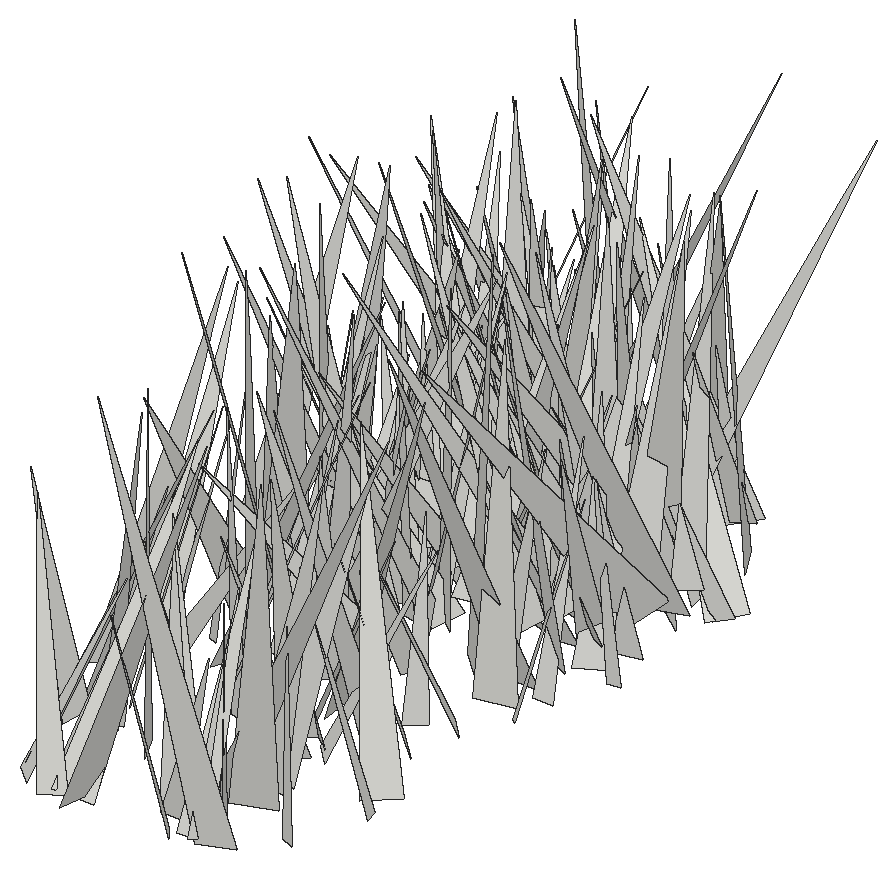
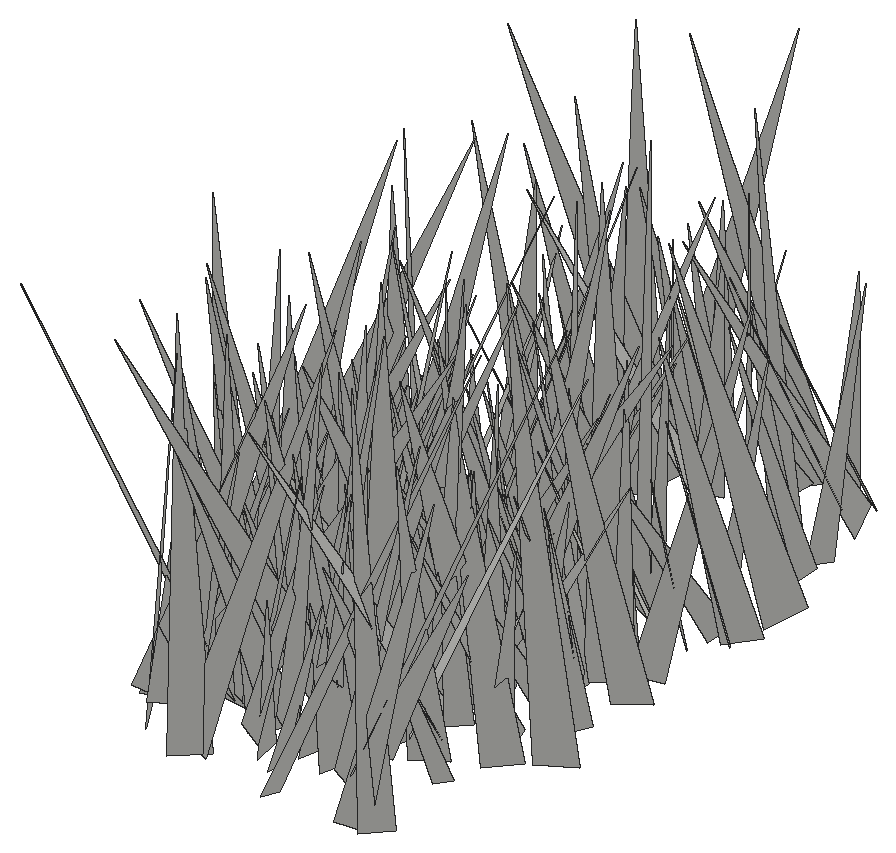
# SketchUp Ruby script. Lengths in inches.
U = 1.inch
M = Sketchup.active_model
def pt(a) = Geom::Point3d.new(a.map { |v| v * U })
def face(e, loops, mat)
  f = e.add_face(loops[0].map { |a| pt(a) })
  loops[1..].each { |l| e.add_face(l.map { |a| pt(a) }).erase! }
  f.material = f.back_material = mat if mat
  f
end
# faces: each face lists its corners as indices into pts; further lists are holes
def faces(e, pts, list, mat = nil) = list.each { |f| face(e, (f[0].is_a?(Array) ? f : [f]).map { |l| l.map { |i| pts[i] } }, mat) }
# xy, xz, yz: faces in a plane at the given z, y or x. An outline is a flat list of corners, or four numbers for a rectangle; further outlines are holes
def ring(l) = l.size == 4 ? [[l[0], l[1]], [l[2], l[1]], [l[2], l[3]], [l[0], l[3]]] : l.each_slice(2).to_a
def flat(e, list, mat, &to3) = list.each { |f| face(e, (f[0].is_a?(Array) ? f : [f]).map { |l| ring(l).map { |u, v| to3.(u, v) } }, mat) }
def xy(e, z, list, mat = nil) = flat(e, list, mat) { |x, y| [x, y, z] }
def xz(e, y, list, mat = nil) = flat(e, list, mat) { |x, z| [x, y, z] }
def yz(e, x, list, mat = nil) = flat(e, list, mat) { |y, z| [x, y, z] }
def lines(e, pts, list) = list.each { |a, b| e.add_line(pt(pts[a]), pt(pts[b])) }
# prism: a flat outline (further loops are holes) pulled along v
def prism(e, loops, v, mat = nil)
  f = face(e, loops, mat); d = Geom::Vector3d.new(v.map { |x| x * U })
  f.pushpull(f.normal.samedirection?(d) ? d.length : -d.length)
end
def box(e, o, s, mat = nil) = prism(e, [[o, [o[0] + s[0], o[1], o[2]], [o[0] + s[0], o[1] + s[1], o[2]], [o[0], o[1] + s[1], o[2]]]], [0, 0, s[2]], mat)
def at(x, y, z, deg = 0) = Geom::Transformation.translation(pt([x, y, z])) * Geom::Transformation.rotation(ORIGIN, Z_AXIS, deg.degrees)
def axes(o, x, y, z) = Geom::Transformation.new([*x, 0, *y, 0, *z, 0, *pt(o).to_a, 1])
def part(name) = M.definitions.add(name)
# library, detail: a bought-in or finely detailed component or shape, given as its bounding box
def library(name, o, s) = part(name).tap { |d| box(d.entities, o, s) }
def detail(e, o, s) = box(e.add_group.entities, o, s)
def put(e, d, t, mat = nil) = e.add_instance(d, t).tap { |i| i.material = mat if mat }
def group(e, t, mat = nil) = e.add_group.tap { |g| g.transformation = t; g.material = mat if mat }.entities
root = M.entities
c1 = part("fur_instance\#9")
p = [[0.8125,0,1.79],[0.67,-0.02,1.48],[0,-0.11,0],[0,0.11,0]]
faces(c1.entities,p,[[0,1,2,3]])
put(root,c1,axes([145.41,167.63,-28.22],[-0.98581,-7.65367,2.64082],[-7.9173,0.35473,-1.92744],[-1.69382,2.79641,7.47232]))
put(root,c1,axes([143.71,167.37,-28.22],[-3.00946,-2.45302,0.73779],[-2.54129,3.00205,-0.38468],[0.32167,0.76736,3.86344]))
put(root,c1,axes([140.13,167.29,-28.22],[7.76844,-0.71206,0.72464],[-0.74639,-7.79129,0.34557],[-0.68922,0.41169,7.79335]))
put(root,c1,axes([143.16,168.27,-28.22],[1.4619,-3.63585,0.57448],[-3.60479,-1.28901,1.01518],[0.74496,0.89757,3.78497]))
put(root,c1,axes([139.28,167.01,-28.22],[-1.32199,4.73147,0.88748],[4.77716,1.17578,0.84759],[-0.59431,-1.0737,4.83901]))
put(root,c1,axes([137.77,167.43,-28.22],[2.47782,3.1575,0.0552],[3.13992,-2.45577,-0.47176],[0.33732,-0.3344,3.98583]))
put(root,c1,axes([142.86,168.82,-28.22],[1.68942,-4.24341,1.91691],[-4.60334,-1.82876,0.00876],[-0.70022,1.78447,4.56734]))
put(root,c1,axes([144.73,167.74,-28.22],[3.50267,-1.34823,2.1537],[-1.97697,-3.75014,0.86764],[-1.59615,1.68627,3.65152]))
put(root,c1,axes([144.74,170.4,-28.22],[3.4393,-6.56896,1.063],[-6.65437,-3.3911,0.57422],[0.02233,1.20797,7.39258]))
put(root,c1,axes([144.92,168.69,-28.22],[3.08289,1.97486,1.70839],[2.08981,-3.45082,0.21788],[-1.56569,-0.71742,3.6547]))
put(root,c1,axes([144.52,167.62,-28.22],[-1.16488,5.07104,1.08343],[5.11451,1.30667,-0.61696],[0.85504,-0.90739,5.16641]))
put(root,c1,axes([138.8,167.92,-28.22],[2.95968,3.81178,0.17357],[3.80838,-2.96454,0.16477],[-0.23661,-0.0359,4.82309]))
put(root,c1,axes([139.86,167.31,-28.22],[-2.51338,5.74575,1.01303],[5.46798,2.70448,-1.77311],[2.03497,-0.17044,6.01555]))
put(root,c1,axes([138.6,170.6,-28.22],[6.91292,1.02767,1.79019],[1.3308,-7.00178,-1.11957],[-1.57792,-1.40299,6.89863]))
put(root,c1,axes([147.02,169.24,-28.22],[1.49909,3.09185,1.25062],[3.12666,-1.78006,0.6529],[-1.16087,-0.8017,3.3735]))
put(root,c1,axes([142.28,170.18,-28.22],[1.59272,-3.9303,2.28796],[-4.37909,-1.9795,-0.352],[-1.22702,1.96293,4.22612]))
put(root,c1,axes([143.78,169.98,-28.22],[7.97011,-1.5942,0.50435],[-1.65185,-7.88792,1.1707],[-0.25934,1.24806,8.04323]))
put(root,c1,axes([136.72,171.46,-28.22],[4.20178,-1.75309,2.00996],[-1.5081,-4.65512,-0.90755],[-2.19975,-0.15714,4.46146]))
put(root,c1,axes([144.19,171.61,-28.22],[1.87666,-6.19619,1.68038],[-6.32701,-1.4881,1.57887],[1.08876,2.03251,6.27868]))
put(root,c1,axes([137.36,168.47,-28.22],[6.20269,2.14266,0.41588],[1.88774,-5.89525,2.21806],[-1.09562,1.97291,6.17613]))
put(root,c1,axes([137.88,171.68,-28.22],[2.52401,-3.24586,0.70539],[-3.32076,-2.44552,0.62916],[0.07602,0.94215,4.0633]))
put(root,c1,axes([139.83,171.2,-28.22],[5.01686,3.02729,2.73746],[3.17963,-5.61852,0.38618],[-2.55892,-1.04628,5.84673]))
put(root,c1,axes([148.0625,172.21,-28.22],[-3.92472,-1.58946,0.29836],[-1.61245,3.78584,-1.04222],[-0.12416,1.07696,4.10409]))
put(root,c1,axes([144.14,172.34,-28.22],[0.67083,5.9533,2.27987],[6.17356,-0.03505,-1.72498],[1.58958,-2.37626,5.73727]))
put(root,c1,axes([136.5625,172.31,-28.22],[4.46137,-0.22154,0.62784],[-0.29219,-4.4737,0.49769],[-0.59824,0.53291,4.43905]))
put(root,c1,axes([143.04,174.73,-28.22],[3.50702,-4.68842,0.88051],[-4.69288,-3.58696,-0.4079],[-0.85643,0.45629,5.84073]))
put(root,c1,axes([141.98,170.6,-28.22],[5.9455,4.2001,0.21568],[4.05072,-5.81939,1.66213],[-1.13095,1.23699,7.08711]))
put(root,c1,axes([144.01,173.83,-28.22],[-1.49858,-3.44059,1.04989],[-3.40031,0.98374,-1.62968],[-1.17382,1.54281,3.38047]))
put(root,c1,axes([137.58,175.24,-28.22],[-3.46561,0.71078,2.1355],[1.4755,3.67824,1.17025],[1.69955,-1.74395,3.33859]))
put(root,c1,axes([147.625,173.29,-28.22],[2.97491,-4.25566,3.74848],[-5.0806,-3.88069,-0.37363],[-2.51977,2.80026,5.17891]))
put(root,c1,axes([145.67,175.61,-28.22],[-0.89834,-6.55906,1.37521],[-6.65422,0.70817,-0.96916],[-0.7961,1.48213,6.54897]))
put(root,c1,axes([137.35,173.47,-28.22],[4.69542,3.0157,0.91715],[3.05189,-4.76105,0.03053],[-0.78841,-0.46959,5.58037]))
put(root,c1,axes([146.1,176.49,-28.22],[-3.15103,-4.03715,0.66571],[-3.75697,3.18756,1.54769],[1.62077,-0.46003,4.88182]))
put(root,c1,axes([140.88,174.49,-28.22],[1.89742,4.59885,2.05217],[4.78177,-2.33318,0.8074],[-1.57969,-1.53878,4.90894]))
put(root,c1,axes([144.35,174.39,-28.22],[3.00056,3.161,0.00616],[3.13284,-2.97269,-0.58633],[0.42105,-0.40809,4.31874]))
put(root,c1,axes([143.93,174.89,-28.22],[-6.33694,-5.31771,1.42218],[-5.44687,5.74429,-2.79146],[-0.79519,3.03026,7.78734]))
put(root,c1,axes([142.93,175.65,-28.22],[3.86213,1.08614,0.2172],[1.09096,-3.86634,-0.0646],[-0.19154,-0.12107,4.01143]))
put(root,c1,axes([142.83,177.24,-28.22],[7.51831,-0.309,0.51299],[-0.23256,-7.46002,-1.08516],[-0.55186,-1.06592,7.446]))
put(root,c1,axes([135.35,174.89,-28.22],[6.60662,-2.19065,2.41659],[-2.83754,-6.55209,1.81792],[-1.6085,2.56075,6.71874]))
put(root,c1,axes([139.13,177.43,-28.22],[-3.84702,-6.56229,2.86732],[-6.71624,4.43571,1.14075],[2.48541,1.82909,7.52076]))
put(root,c1,axes([141.31,176.01,-28.22],[2.64561,4.33348,1.24236],[4.47199,-2.70465,-0.08904],[-0.56902,-1.10798,5.07645]))
put(root,c1,axes([146.58,178.38,-28.22],[-3.28468,-3.33783,0.1825],[-3.30088,3.27904,0.56182],[0.52783,-0.26523,4.64915]))
put(root,c1,axes([141.5,178.35,-28.22],[3.06125,-3.87557,0.82155],[-3.90702,-3.12527,-0.1848],[-0.65588,0.52812,4.93529]))
put(root,c1,axes([142.17,180.51,-28.22],[-5.57045,-1.42182,0.3414],[-1.0257,4.7578,3.07884],[1.04215,-2.91715,4.85512]))
put(root,c1,axes([136.34,180.7,-28.22],[5.34512,-3.23236,0.64666],[-2.65449,-4.95104,-2.80671],[-1.95449,-2.11559,5.5804]))
put(root,c1,axes([135.875,177.12,-28.22],[2.95956,2.83712,0.75066],[2.89518,-2.997,-0.08741],[-0.48027,-0.58351,4.09885]))
put(root,c1,axes([145.45,177.71,-28.22],[-2.47,2.58512,1.49197],[2.74392,2.72878,-0.18549],[1.17462,-0.93843,3.57063]))
put(root,c1,axes([136.35,176.99,-28.22],[3.53802,-1.77872,0.68161],[-1.86523,-2.94336,2.00089],[0.38644,2.07817,3.41729]))
put(root,c1,axes([135.49,176.93,-28.22],[-3.09006,5.24053,1.65653],[5.13422,3.43055,-1.27548],[1.9614,-0.72379,5.94851]))
put(root,c1,axes([146.27,181.89,-28.22],[-0.28609,-7.90952,0.17476],[-7.91116,0.28452,-0.07401],[-0.06767,0.17732,7.91434]))
put(root,c1,axes([138.21,177.04,-28.22],[6.82155,0.82248,0.97272],[0.53436,-6.65794,1.88216],[-1.15634,1.77527,6.60814]))
put(root,c1,axes([142.74,181.92,-27.1],[-6.5639,-4.29471,0.69968],[-4.06333,6.50273,1.7952],[1.55674,-1.13527,7.63588]))
put(root,c1,axes([140.64,179.44,-28.22],[6.1687,-0.67373,2.21616],[-0.70194,-6.55164,-0.0379],[-2.20738,0.2006,6.20527]))
put(root,c1,axes([137.01,177.98,-28.22],[2.28996,3.33239,0.84649],[3.03653,-2.43723,1.38011],[-1.61271,0.14282,3.80053]))
put(root,c1,axes([137.1,181.5,-28.22],[5.72891,-5.77899,0.7373],[-5.79412,-5.75966,-0.12335],[-0.60698,0.43635,8.13646]))
put(root,c1,axes([138.19,177.99,-28.22],[3.1839,3.43631,0.24845],[3.39454,-3.18669,0.57383],[-0.5891,0.20968,4.64932]))
put(root,c1,axes([139.12,181.21,-28.22],[2.70621,-3.86796,1.26709],[-3.69816,-2.97221,-1.17466],[-1.70008,0.30833,4.57219]))
put(root,c1,axes([146.53,180.4,-28.22],[-1.49682,6.02983,3.22428],[6.74332,1.8484,-0.32627],[1.1325,-3.03643,6.20426]))
put(root,c1,axes([139.68,180.76,-28.22],[3.87779,-2.1954,0.31482],[-2.2129,-3.78759,0.8446],[0.14815,0.88911,4.37535]))
put(root,c1,axes([143.24,180.38,-28.22],[-3.36679,-6.63148,1.92496],[-6.20382,1.96447,-4.08298],[-3.03226,3.34389,6.21619]))
put(root,c1,axes([138.88,181.55,-27.1],[6.72646,1.81373,2.96578],[2.30607,-7.16166,-0.85049],[-2.60144,-1.65881,6.91459]))
put(root,c1,axes([144.71,181.58,-28.22],[-4.52397,-6.09316,3.51067],[-6.34353,5.33763,1.08955],[3.03497,2.07386,7.51038]))
put(root,c1,axes([140.73,181.74,-28.22],[-7.80525,1.8691,2.4402],[2.24771,8.01322,1.05174],[2.09664,-1.63243,7.95672]))
put(root,c1,axes([139.53,178.46,-28.22],[1.84381,6.83005,0.32521],[6.75707,-1.87158,0.99709],[-1.04756,-0.05069,7.00393]))
put(root,c1,axes([148.02,186.2,-27.1],[5.96387,-5.74764,0.45925],[-4.68382,-5.21453,-4.43673],[-3.36276,-2.93042,6.99418]))
put(root,c1,axes([137.58,182.1875,-28.22],[5.69454,1.71793,1.14191],[1.95584,-5.5622,-1.38552],[-0.6557,-1.67144,5.78441]))
put(root,c1,axes([147.72,179.86,-28.22],[2.63979,2.66437,0.28601],[2.37928,-2.51517,1.47039],[-1.23275,0.85099,3.4504]))
put(root,c1,axes([135.31,183.23,-27.1],[5.21183,-0.69159,1.00189],[-0.40075,-5.13378,-1.45906],[-1.14955,-1.3458,5.051]))
put(root,c1,axes([136.49,181.375,-27.1],[3.11612,2.14822,0.04863],[2.13222,-3.08072,-0.53874],[0.26618,-0.47091,3.74631]))
put(root,c1,axes([145.86,181.5,-28.22],[3.92282,-1.4058,1.44453],[-1.66907,-4.03753,0.60333],[-1.1301,1.0833,4.1232]))
put(root,c1,axes([147.85,181.91,-27.1],[-3.61019,-4.99925,2.09321],[-5.40705,3.49453,-0.97958],[0.37125,2.28107,6.08822]))
put(root,c1,axes([144.81,185.4,-27.1],[-6.99156,-3.62516,0.34789],[-3.32905,6.6672,2.57109],[1.47657,-2.13338,7.444]))
put(root,c1,axes([141.02,186.1,-28.22],[-5.60645,-3.595,0.79099],[-2.74257,5.04084,3.47133],[2.4552,-2.57833,5.68385]))
put(root,c1,axes([139.18,183.02,-28.22],[3.73633,3.15118,1.53756],[3.50493,-3.41917,-1.50964],[-0.09758,-2.15258,4.64878]))
put(root,c1,axes([142.04,183.64,-28.22],[-4.08347,2.98679,1.40676],[3.27171,3.36098,2.36101],[-0.44252,-2.71247,4.47451]))
put(root,c1,axes([142.17,181.43,-27.1],[2.11114,4.26728,1.69749],[4.08085,-2.60007,1.46097],[-2.10662,-0.76029,4.53125]))
put(root,c1,axes([147.66,181.41,-28.22],[0.78964,4.34465,0.57519],[4.335,-0.86018,0.54605],[-0.64386,-0.46311,4.38193]))
put(root,c1,axes([147,184.85,-28.22],[4.67947,-2.49587,0.44393],[-2.29207,-4.56374,-1.49753],[-1.08298,-1.12554,5.08765]))
put(root,c1,axes([138.2,182.58,-28.22],[1.93796,6.92662,2.2466],[6.80944,-0.90011,-3.09877],[2.58009,-2.82714,6.49087]))
put(root,c1,axes([141.64,183.25,-27.1],[5.91305,2.63208,1.30513],[2.84881,-5.85376,-1.10147],[-0.71801,-1.54954,6.37799]))
put(root,c1,axes([141.88,183.62,-28.22],[-3.26006,-5.04679,2.60885],[-5.29814,3.78652,0.70434],[2.05082,1.75965,5.96674]))
put(root,c1,axes([147.875,183.93,-27.1],[-2.11494,-3.26023,0.3236],[-3.25153,2.04149,-0.68318],[-0.40176,0.64034,3.82562]))
put(root,c1,axes([138.71,183.23,-27.1],[4.6292,0.17151,0.50537],[0.17521,-4.6565,-0.02456],[-0.5041,-0.0434,4.63231]))
put(root,c1,axes([140.17,183.61,-28.22],[-0.67807,6.71445,3.30984],[6.96597,-0.65101,2.74773],[-2.74118,-3.31527,6.16389]))
put(root,c1,axes([139.07,182.91,-27.1],[-0.2633,5.21725,2.01289],[5.21535,0.95622,-1.79623],[2.01778,-1.79073,4.90536]))
put(root,c1,axes([145.99,184.87,-28.22],[-0.56318,-3.80765,0.20803],[-3.75255,0.51599,-0.71463],[-0.67806,0.30692,3.78215]))
put(root,c1,axes([145.59,183.31,-27.1],[-7.05219,-0.0174,0.36445],[-0.04272,7.04446,-0.49029],[0.36236,0.49184,7.03515]))
put(root,c1,axes([144.85,185.38,-28.22],[-1.82356,-4.42835,0.39133],[-4.41286,1.85435,0.42054],[0.53859,0.19978,4.77062]))
put(root,c1,axes([138.22,186.54,-27.1],[-4.13321,-3.41194,0.20507],[-3.07913,3.85633,2.10107],[1.48403,-1.5014,4.93054]))
put(root,c1,axes([138.97,183.04,-28.22],[-1.4583,4.1794,0.64732],[4.14586,1.27741,1.09233],[-0.83566,-0.95598,4.28962]))
put(root,c1,axes([148.3125,186.86,-27.1],[0.33917,-8.30019,0.61155],[-8.21231,-0.43312,-1.32383],[-1.35096,0.54903,8.20095]))
put(root,c1,axes([138.89,184.26,-27.1],[-3.23089,-3.2407,0.20186],[-3.09319,2.98531,-1.58167],[-0.98745,1.25194,4.29408]))
put(root,c1,axes([134.44,183.81,-27.1],[1.86303,-6.4471,2.90273],[-6.99316,-1.23765,1.73947],[1.04242,3.21946,6.48153]))
put(root,c1,axes([146.71,184.92,-27.1],[-2.94659,-4.28728,0.79485],[-4.35538,2.84813,-0.78348],[-0.2081,1.09651,5.14289]))
put(root,c1,axes([148.76,183.63,-28.22],[0.66208,3.60921,1.19442],[3.54519,-1.02396,1.12897],[-1.37285,-0.90361,3.49144]))
put(root,c1,axes([145.33,186.25,-28.22],[0.2783,-5.0487,0.14304],[-4.93686,-0.24166,1.07529],[1.0664,0.19877,4.94071]))
put(root,c1,axes([135.93,184.55,-28.22],[3.08181,-1.73974,0.98019],[-1.88437,-3.1302,0.36886],[-0.66077,0.81254,3.51969]))
put(root,c1,axes([136.61,183.62,-27.1],[2.93854,2.24557,1.05284],[2.03507,-3.11619,0.96641],[-1.41759,0.18132,3.56983]))
put(root,c1,axes([137.88,183.38,-28.22],[-2.24412,3.20659,0.81725],[3.00578,2.38826,-1.11699],[1.38398,0.01256,3.75108]))
put(root,c1,axes([145.97,184.78,-27.1],[-4.77809,0.40303,0.49366],[0.4272,4.79644,0.21897],[0.47289,-0.2608,4.79006]))
put(root,c1,axes([145.02,184.375,-27.1],[2.48119,3.58815,0.88423],[3.68479,-2.32113,-0.92071],[0.2811,-1.24521,4.2642]))
put(root,c1,axes([147.78,185.37,-28.22],[-0.62718,-6.98929,2.39617],[-7.29856,0.2117,-1.29283],[-1.15016,2.46782,6.89725]))
put(root,c1,axes([146.04,186.73,-27.1],[2.95419,-3.46444,1.08183],[-2.95275,-3.10527,-1.88109],[-2.11044,-0.50488,4.14621]))
put(root,c1,axes([139.31,184.8,-27.1],[1.67153,-3.68103,1.97281],[-4.08391,-1.88531,-0.05752],[-0.87388,1.76964,4.04237]))
put(root,c1,axes([146.81,185.04,-28.22],[-2.61332,3.50076,2.27341],[3.90248,3.00092,-0.13507],[1.48133,-1.72983,4.36652]))
put(root,c1,axes([144.45,185.12,-28.22],[-5.1387,-6.17044,1.38685],[-6.22365,4.61615,-2.52214],[-1.12419,2.64967,7.62361]))
put(root,c1,axes([136.89,183.61,-27.1],[1.45638,3.8911,0.37542],[3.87774,-1.48869,0.38679],[-0.49475,-0.21394,4.13668]))
put(root,c1,axes([138.44,185.96,-27.1],[0.50859,-3.54434,0.97529],[-3.61365,-0.30136,0.78924],[0.67458,1.05784,3.49258]))
put(root,c1,axes([142.53,186.91,-28.22],[-1.81224,-5.34948,0.90018],[-5.42401,1.80193,-0.21131],[0.08596,0.92064,5.64415]))
put(root,c1,axes([135.71,186.62,-27.1],[0.50493,-3.90237,0.56248],[-3.75126,-0.30094,1.27958],[1.21364,0.69337,3.72104]))
put(root,c1,axes([135.07,186.87,-28.22],[1.45469,-7.67033,1.86376],[-7.74266,-1.0178,1.85445],[1.53584,2.13396,7.5836]))
put(root,c1,axes([140.71,184.6,-28.22],[0.94432,5.62245,1.27282],[5.76049,-0.87093,-0.42662],[0.22085,-1.32412,5.68522]))
put(root,c1,axes([142.125,186.1,-27.1],[6.74375,-1.56753,0.95704],[-1.61805,-6.79399,0.27364],[-0.86892,0.48558,6.91813]))
put(root,c1,axes([140.84,184.57,-27.1],[1.32341,3.79294,0.4756],[3.74321,-1.38791,0.65276],[-0.77522,-0.22654,3.9638]))
put(root,c1,axes([144.5625,187.7,-28.22],[-6.28485,-0.79991,0.77187],[-0.56549,6.11624,1.73401],[0.95701,-1.63912,6.09364]))
put(root,c1,axes([142.03,188.2,-27.1],[-4.79038,-5.44103,1.36632],[-5.2062,4.98101,1.5825],[2.08977,-0.06337,7.07448]))
put(root,c1,axes([146.2,189.93,-28.22],[4.16443,-6.48584,0.7003],[-5.50995,-3.94185,-3.74183],[-3.49241,-1.51483,6.7385]))
put(root,c1,axes([139.47,185.77,-28.22],[3.42061,-2.16163,2.16053],[-2.46149,-3.8706,0.02453],[-1.81151,1.17767,4.04631]))
put(root,c1,axes([144,186.23,-27.1],[0.99186,4.25892,2.03749],[4.71935,-0.95274,-0.30591],[-0.13232,-2.05608,4.36218]))
put(root,c1,axes([141.59,185.3,-27.1],[-4.74257,5.72398,1.5327],[5.90767,4.72004,0.65254],[0.46105,-1.60076,7.40474]))
put(root,c1,axes([147.55,184,-28.22],[-5.09281,3.29268,0.78292],[3.01884,5.05892,-1.63872],[1.53013,0.9783,5.83893]))
put(root,c1,axes([147.62,188.18,-28.22],[-3.80651,-3.12707,0.03174],[-3.06593,3.74155,0.93273],[0.61617,-0.70095,4.83716]))
put(root,c1,axes([143.11,183.5,-27.1],[-4.70627,4.28235,1.06672],[3.70191,4.67966,-2.45399],[2.40255,1.178,5.87073]))
put(root,c1,axes([142.11,185.5625,-28.22],[-1.29453,3.3269,0.92168],[3.25121,1.50588,-0.8692],[1.16077,-0.50757,3.46245]))
put(root,c1,axes([136.4,187.91,-28.22],[2.49015,-6.48815,0.76577],[-6.33726,-2.19962,1.97082],[1.58797,1.39602,6.66429]))
put(root,c1,axes([136.97,185.32,-27.1],[0.32449,4.79651,0.65441],[4.29347,0.01783,-2.25961],[2.23626,-0.73022,4.24334]))
put(root,c1,axes([139.54,187.36,-28.22],[-7.27615,-1.41209,3.18772],[-1.2687,7.94356,0.62294],[3.24745,-0.06052,7.38568]))
put(root,c1,axes([137.87,188.32,-27.1],[2.72527,-3.47225,0.02549],[-3.46346,-2.7159,0.33551],[0.24824,0.22715,4.40125]))
put(root,c1,axes([144.92,187.79,-27.1],[3.71508,-1.29272,0.27873],[-1.28155,-3.72443,-0.19222],[-0.32626,-0.0905,3.92887]))
put(root,c1,axes([137.1875,187.13,-28.22],[-2.21806,2.84038,1.31516],[3.07662,2.27502,0.2754],[0.57601,-1.21396,3.59328]))
put(root,c1,axes([137.1,186.25,-28.22],[4.11341,0.99659,0.14821],[0.94897,-4.04143,0.83763],[-0.33855,0.78037,4.1487]))
put(root,c1,axes([142.34,184.64,-28.22],[5.39727,3.08007,0.18691],[2.81936,-5.07536,2.22356],[-1.25418,1.84558,5.80286]))
put(root,c1,axes([145.99,189.2,-27.1],[2.29516,-7.21123,1.1617],[-7.23425,-2.07612,1.40519],[1.00849,1.5189,7.43607]))
put(root,c1,axes([139.01,189.34,-27.1],[-5.75391,-4.14909,0.07824],[-4.14913,5.75437,0.02082],[0.07564,0.02888,7.0938]))
put(root,c1,axes([139.53,185.22,-27.1],[-5.90287,3.96424,1.22936],[3.5461,5.92766,-2.08769],[2.15678,1.10365,6.7971]))
put(root,c1,axes([144.73,189.82,-28.22],[-0.95701,-7.3765,1.52863],[-7.35851,1.24531,1.40248],[1.61303,1.30453,7.30491]))
put(root,c1,axes([141.4,189.49,-27.1],[2.7716,-4.32676,0.73791],[-4.29866,-2.85215,-0.57784],[-0.88707,0.30254,5.10575]))
put(root,c1,axes([144.55,188.4,-27.1],[-1.98157,5.41612,3.08152],[6.10168,2.34277,-0.19399],[1.26474,-2.81671,5.76397]))
put(root,c1,axes([145.84,189.64,-28.22],[-0.88156,-7.55851,1.51866],[-6.98391,0.13553,-3.37952],[-3.26533,1.75074,6.81814]))
put(root,c1,axes([144.51,187.16,-27.1],[0.16131,6.95669,2.04491],[7.08472,0.28432,-1.5261],[1.54396,-2.03146,6.78915]))
put(root,c1,axes([146.39,187.58,-27.1],[-1.99924,6.11191,2.2816],[6.3463,2.375,-0.80119],[1.51181,-1.88733,6.38047]))
put(root,c1,axes([141.53,190.79,-28.22],[0.11863,-7.1905,0.64579],[-7.08435,-0.24031,-1.37429],[-1.39009,0.61104,7.05894]))
put(root,c1,axes([140.8,188.4,-27.1],[5.17413,-4.7343,3.23528],[-5.24163,-5.67192,0.08293],[-2.32507,2.25121,7.01272]))
put(root,c1,axes([143.2,188.49,-27.1],[-4.86777,3.35697,1.6535],[3.6105,4.92638,0.62739],[0.98366,-1.46972,5.8797]))
put(root,c1,axes([148.85,189.1,-28.22],[-0.30638,-3.92044,1.36874],[-3.76361,-0.31774,-1.75256],[-1.75458,1.36615,3.52026]))
put(root,c1,axes([138.49,192.77,-27.1],[-6.95908,-3.88864,0.42907],[-3.38575,6.42493,3.31533],[1.96017,-2.70799,7.24975]))
put(root,c1,axes([140.65,190.56,-27.1],[4.51111,-4.76568,1.07484],[-4.75985,-4.61702,-0.49408],[-1.1004,0.43419,6.54353]))
put(root,c1,axes([147.36,189.84,-28.22],[-5.30182,-0.75056,0.88287],[-0.65483,5.35184,0.61739],[0.95603,-0.49663,5.31898]))
put(root,c1,axes([143.37,188.29,-28.22],[-7.85501,-1.13743,1.66782],[-1.3997,7.89692,-1.20666],[1.45472,1.45652,7.84468]))
put(root,c1,axes([143.24,190,-27.1],[3.93197,-0.07434,1.3447],[0.21137,-4.06439,-0.84276],[-1.33006,-0.86567,3.84131]))
put(root,c1,axes([144.75,187.49,-28.22],[7.43701,2.08557,1.03262],[1.85087,-7.39668,1.60887],[-1.41074,1.29018,7.55449]))
put(root,c1,axes([144.43,187.83,-28.22],[-6.83852,1.49302,2.47832],[0.97247,7.17644,-1.63995],[2.72497,1.18576,6.80477]))
put(root,c1,axes([143.68,190.78,-28.22],[3.60736,-4.41491,0.21347],[-4.38405,-3.53869,0.89879],[0.56311,0.73233,5.62998]))
put(root,c1,axes([146.99,188.58,-27.1],[-6.72767,0.28008,1.7782],[-0.11729,6.79671,-1.51427],[1.7963,1.49276,6.56102]))
put(root,c1,axes([137.23,189.91,-28.22],[0.91676,-3.52562,1.5814],[-3.59518,-0.18259,1.67709],[1.41617,1.81877,3.23385]))
put(root,c1,axes([143.32,189.11,-27.1],[3.71678,-0.58843,1.31141],[-0.99782,-3.67326,1.17982],[-1.0346,1.42876,3.57333]))
put(root,c1,axes([140.33,189.71,-28.22],[-2.24155,-3.80564,2.54295],[-4.42537,2.52493,-0.12217],[1.16862,2.26183,4.41503]))
put(root,c1,axes([148.85,189.28,-28.22],[-3.95209,5.35159,0.47213],[5.26841,3.74586,1.6413],[-1.05182,-1.34553,6.44707]))
put(root,c1,axes([138.4375,189.12,-28.22],[-2.92394,5.35838,1.35906],[5.44647,3.05552,-0.32925],[0.94614,-1.02969,6.09534]))
put(root,c1,axes([147.98,188.35,-27.1],[-6.09704,1.94582,1.05535],[1.61207,6.02238,-1.79053],[1.51697,1.42075,6.14444]))
put(root,c1,axes([141.01,193.96,-28.22],[-7.53778,-2.79862,0.78068],[-2.32716,7.11502,3.03655],[1.73954,-2.60846,7.44512]))
put(root,c1,axes([147.14,191.15,-27.1],[-3.57828,-1.18752,0.86435],[-1.11493,3.67791,0.43741],[0.95617,-0.15551,3.74473]))
put(root,c1,axes([139.8,191.76,-28.22],[-2.71876,-5.31687,1.33657],[-5.469,2.73415,-0.24823],[0.3815,1.3048,5.9665]))
put(root,c1,axes([139.83,188.69,-28.22],[-3.50119,3.09472,0.56001],[2.74674,3.41714,-1.71109],[1.53177,0.94611,4.34831]))
put(root,c1,axes([140.42,191.17,-28.22],[6.63487,-1.65212,1.91106],[-1.73662,-6.8834,0.0785],[-1.83462,0.54083,6.83702]))
put(root,c1,axes([142.92,188.87,-27.1],[-3.90742,5.66938,0.63215],[5.60395,3.95813,-0.85923],[1.06639,-0.02677,6.83166]))
put(root,c1,axes([141.61,191.06,-28.22],[-4.97089,0.8761,1.32855],[0.91857,5.13772,0.0489],[1.29955,-0.28038,5.04727]))
put(root,c1,axes([141.59,190.3,-28.22],[-3.26703,2.9675,0.38966],[2.97957,3.27925,0.00816],[0.28293,-0.26806,4.41355]))
put(root,c1,axes([146.64,192.85,-27.1],[1.6071,-3.85332,0.26864],[-3.82652,-1.62792,-0.45895],[-0.52725,0.06941,4.14972]))
put(root,c1,axes([136.86,193.75,-28.22],[6.92696,-1.79403,0.01467],[-1.72828,-6.68834,-1.86567],[-0.48147,-1.80253,6.90801]))
put(root,c1,axes([146.5625,192.8,-27.1],[1.94153,-7.03493,2.68991],[-6.84514,-2.80689,-2.40016],[-3.14163,1.7682,6.89195]))
put(root,c1,axes([141.46,190.11,-28.22],[0.8824,6.11345,1.2337],[6.18895,-1.01221,0.58924],[-0.77016,-1.12963,6.14863]))
put(root,c1,axes([138.73,191.36,-27.1],[-2.74524,3.88345,0.46197],[3.73915,2.44095,1.70042],[-1.14601,-1.33847,4.4414]))
put(root,c1,axes([137.6875,194,-28.22],[1.38462,-5.25865,0.1546],[-5.22749,-1.39323,-0.57157],[-0.5921,0.00308,5.40776]))
put(root,c1,axes([138.39,188.39,-27.1],[6.17595,4.1917,0.11311],[3.92557,-5.85042,2.46738],[-1.47413,1.98185,7.04448]))
put(root,c1,axes([145.65,192.07,-27.1],[-2.59622,-3.87524,1.56211],[-4.17566,2.47102,-0.8099],[0.14666,1.75346,4.59368]))
put(root,c1,axes([142.77,191.27,-27.1],[4.39475,-2.24157,1.41228],[-2.61052,-4.13054,1.56743],[-0.4521,2.06082,4.67778]))
put(root,c1,axes([146.18,193.09,-27.1],[2.32734,-2.83374,0.7234],[-2.82694,-2.41664,-0.37171],[-0.74954,0.31569,3.64807]))
put(root,c1,axes([147.125,192.48,-28.22],[-5.46396,-3.21591,2.3792],[-3.43589,5.83542,-0.00311],[2.04873,1.20967,6.3401]))
put(root,c1,axes([142.69,192.9,-27.1],[-2.18314,-4.32344,1.23175],[-4.48368,1.99494,-0.94459],[-0.32548,1.51774,4.75036]))
put(root,c1,axes([143.6875,194.55,-27.1],[-2.92587,-7.18113,1.16279],[-7.26033,2.80394,-0.95233],[-0.45638,1.43204,7.69561]))
put(root,c1,axes([144.07,190.77,-27.1],[-6.55777,-1.69063,0.96933],[-1.94723,5.82112,-3.02077],[0.07829,3.17151,6.06115]))
put(root,c1,axes([143.35,195.1,-27.1],[6.03142,-3.81553,0.06105],[-3.78285,-5.99326,-0.84318],[-0.50203,-0.68018,7.08699]))
put(root,c1,axes([141.83,192.09,-27.1],[3.01287,6.59159,3.14785],[6.68601,-3.85992,1.68335],[-2.94198,-2.02171,7.04931]))
put(root,c1,axes([141.3,190.01,-27.1],[8.13391,1.72844,0.70897],[1.41113,-7.75982,2.72846],[-1.22428,2.53935,7.85515]))
put(root,c1,axes([144.98,191.24,-27.1],[4.52009,6.67395,0.30614],[6.59904,-4.40227,-1.46264],[1.04307,-1.07006,7.92676]))
put(root,c1,axes([141.95,192.35,-28.22],[-3.96056,0.86775,0.15545],[0.85071,3.94968,-0.37345],[0.23119,0.33194,4.03727]))
put(root,c1,axes([142.84,191.84,-28.22],[-3.9297,0.38452,0.60241],[0.18265,3.7953,-1.23109],[0.69093,1.18368,3.75164]))
